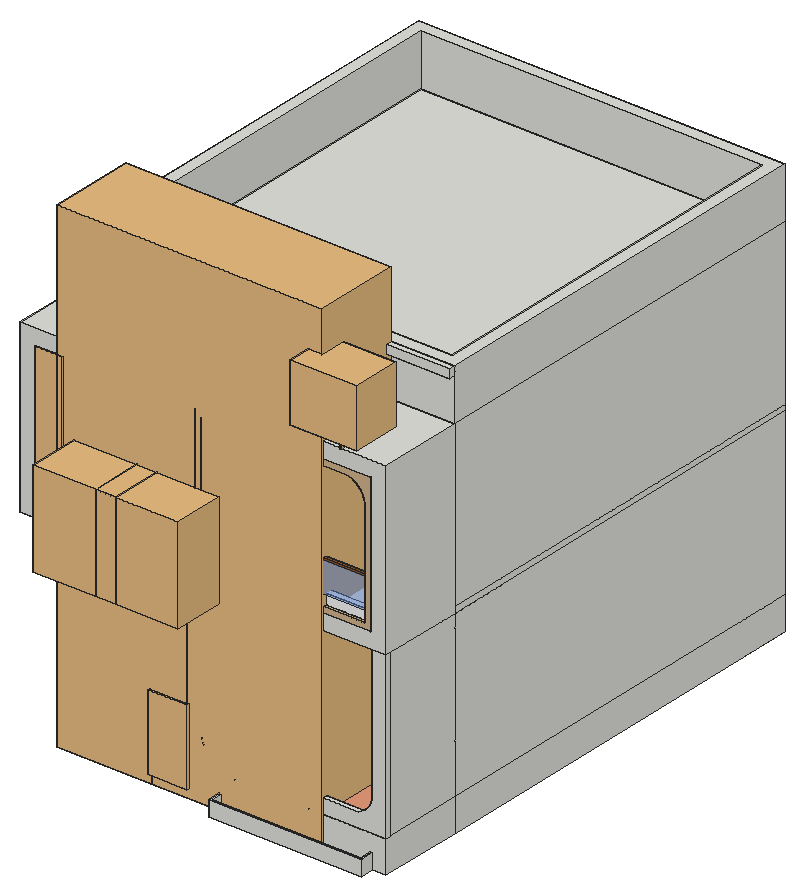
# SketchUp Ruby script. Lengths in inches.
U = 1.inch
M = Sketchup.active_model
def pt(a) = Geom::Point3d.new(a.map { |v| v * U })
def face(e, loops, mat)
  f = e.add_face(loops[0].map { |a| pt(a) })
  loops[1..].each { |l| e.add_face(l.map { |a| pt(a) }).erase! }
  f.material = f.back_material = mat if mat
  f
end
# faces: each face lists its corners as indices into pts; further lists are holes
def faces(e, pts, list, mat = nil) = list.each { |f| face(e, (f[0].is_a?(Array) ? f : [f]).map { |l| l.map { |i| pts[i] } }, mat) }
# xy, xz, yz: faces in a plane at the given z, y or x. An outline is a flat list of corners, or four numbers for a rectangle; further outlines are holes
def ring(l) = l.size == 4 ? [[l[0], l[1]], [l[2], l[1]], [l[2], l[3]], [l[0], l[3]]] : l.each_slice(2).to_a
def flat(e, list, mat, &to3) = list.each { |f| face(e, (f[0].is_a?(Array) ? f : [f]).map { |l| ring(l).map { |u, v| to3.(u, v) } }, mat) }
def xy(e, z, list, mat = nil) = flat(e, list, mat) { |x, y| [x, y, z] }
def xz(e, y, list, mat = nil) = flat(e, list, mat) { |x, z| [x, y, z] }
def yz(e, x, list, mat = nil) = flat(e, list, mat) { |y, z| [x, y, z] }
def lines(e, pts, list) = list.each { |a, b| e.add_line(pt(pts[a]), pt(pts[b])) }
# prism: a flat outline (further loops are holes) pulled along v
def prism(e, loops, v, mat = nil)
  f = face(e, loops, mat); d = Geom::Vector3d.new(v.map { |x| x * U })
  f.pushpull(f.normal.samedirection?(d) ? d.length : -d.length)
end
def box(e, o, s, mat = nil) = prism(e, [[o, [o[0] + s[0], o[1], o[2]], [o[0] + s[0], o[1] + s[1], o[2]], [o[0], o[1] + s[1], o[2]]]], [0, 0, s[2]], mat)
def at(x, y, z, deg = 0) = Geom::Transformation.translation(pt([x, y, z])) * Geom::Transformation.rotation(ORIGIN, Z_AXIS, deg.degrees)
def axes(o, x, y, z) = Geom::Transformation.new([*x, 0, *y, 0, *z, 0, *pt(o).to_a, 1])
def part(name) = M.definitions.add(name)
# library, detail: a bought-in or finely detailed component or shape, given as its bounding box
def library(name, o, s) = part(name).tap { |d| box(d.entities, o, s) }
def detail(e, o, s) = box(e.add_group.entities, o, s)
def put(e, d, t, mat = nil) = e.add_instance(d, t).tap { |i| i.material = mat if mat }
def group(e, t, mat = nil) = e.add_group.tap { |g| g.transformation = t; g.material = mat if mat }.entities
root = M.entities
M.materials.add("Heather_Skin").color = [229, 155, 121]
M.materials.add("[0035_Tan]").color = [210, 180, 140]
M.materials.add("[0128_White]").color = [255, 255, 255]
M.materials["[0128_White]"].alpha = 0.85
M.materials.add("[0129_WhiteSmoke]").color = [245, 245, 245]
M.materials.add("[Color M09]").color = [0, 0, 0]
M.materials.add("[Translucent Glass Blue]").color = [100, 149, 237]
M.materials["[Translucent Glass Blue]"].alpha = 0.5
M.materials.add("[Wood Cherry Original]").color = [152, 86, 42]
c1 = library("Rose+Jali+Design",[0,0,0],[20,1,36])
c2 = library("Hanging plant cluster",[-9.08,-12.96,-0.71],[50.92,60.22,69.94])
c3 = library("Door+01",[0,-2.84,-4],[33.31,7.1,94])
c4 = library("Window with transom",[0,0,0],[5.2,55.12,70.87])
c5 = part("Divided light sash")
xy(c5.entities,0,[[[0,-7,18,20],[1,-5,17,19]]])
xy(c5.entities,0.25,[[8.75,-5,8.75,6.75,1,6.75,1,7.25,8.75,7.25,8.75,19,9.25,19,9.25,7.25,17,7.25,17,6.75,9.25,6.75,9.25,-5]])
xy(c5.entities,0.5,[[1,-5,8.75,6.75],[9.25,-5,17,6.75],[1,7.25,8.75,19],[9.25,7.25,17,19]])
xy(c5.entities,0.75,[[8.75,-5,9.25,-5,9.25,6.75,17,6.75,17,7.25,9.25,7.25,9.25,19,8.75,19,8.75,7.25,1,7.25,1,6.75,8.75,6.75]])
xy(c5.entities,1,[[[0,-7,18,20],[1,-5,17,19]]])
xz(c5.entities,-7,[[0,0,18,1]])
xz(c5.entities,-5,[[1,0,1,0.5,8.75,0.5,8.75,0.25,9.25,0.25,9.25,0.5,17,0.5,17,0],[8.75,0.25,9.25,0.75],[1,0.5,1,1,17,1,17,0.5,9.25,0.5,9.25,0.75,8.75,0.75,8.75,0.5]])
xz(c5.entities,6.75,[[1,0.25,8.75,0.5],[9.25,0.25,17,0.5],[1,0.5,8.75,0.75],[9.25,0.5,17,0.75]])
xz(c5.entities,7.25,[[1,0.25,8.75,0.5],[9.25,0.25,17,0.5],[1,0.5,8.75,0.75],[9.25,0.5,17,0.75]])
xz(c5.entities,19,[[1,0,17,0,17,0.5,9.25,0.5,9.25,0.25,8.75,0.25,8.75,0.5,1,0.5],[8.75,0.25,9.25,0.75],[1,0.5,8.75,0.5,8.75,0.75,9.25,0.75,9.25,0.5,17,0.5,17,1,1,1]])
xz(c5.entities,20,[[0,0,18,1]])
yz(c5.entities,0,[[-7,0,20,1]])
yz(c5.entities,1,[[-5,0,19,0,19,0.5,7.25,0.5,7.25,0.25,6.75,0.25,6.75,0.5,-5,0.5],[6.75,0.25,7.25,0.75],[-5,0.5,6.75,0.5,6.75,0.75,7.25,0.75,7.25,0.5,19,0.5,19,1,-5,1]])
yz(c5.entities,8.75,[[-5,0.25,6.75,0.5],[7.25,0.25,19,0.5],[-5,0.5,6.75,0.75],[7.25,0.5,19,0.75]])
yz(c5.entities,9.25,[[-5,0.25,6.75,0.5],[7.25,0.25,19,0.5],[-5,0.5,6.75,0.75],[7.25,0.5,19,0.75]])
yz(c5.entities,17,[[-5,0,-5,0.5,6.75,0.5,6.75,0.25,7.25,0.25,7.25,0.5,19,0.5,19,0],[6.75,0.25,7.25,0.75],[-5,0.5,-5,1,19,1,19,0.5,7.25,0.5,7.25,0.75,6.75,0.75,6.75,0.5]])
yz(c5.entities,18,[[-7,0,20,1]])
c6 = part("Double-hung window 69 in. x 58 in. triple row with mullions")
xy(c6.entities,-2.625,[[[1.5,1.5,60.5,56.5],[22,2.5,40,55.5],[2.5,2.5,20.5,55.5],[41.5,2.5,59.5,55.5]]])
xy(c6.entities,0,[[[0,0,62,58],[1.5,1.5,60.5,56.5]],[1.5,1.5,60.5,2.5],[1.5,2.5,2,2.5,2,56,60,56,60,2.5,60.5,2.5,60.5,56.5,1.5,56.5],[21,2.5,21.5,56],[40.5,2.5,41,56]])
xy(c6.entities,1,[[[0,0,62,58],[1.5,2,60.5,56.5]]])
xz(c6.entities,0,[[0,0,62,1]])
xz(c6.entities,1.5,[[1.5,-2.625,60.5,0]])
xz(c6.entities,2.5,[[2.5,-2.625,2.5,-0.5,2,0,21,0,20.5,-0.5,20.5,-2.625],[22,-2.625,22,-0.5,21.5,0,40.5,0,40,-0.5,40,-2.625],[41.5,-2.625,41.5,-0.5,41,0,60,0,59.5,-0.5,59.5,-2.625]])
xz(c6.entities,55.5,[[2.5,-2.625,20.5,-0.5],[22,-2.625,40,-0.5],[41.5,-2.625,59.5,-0.5]])
xz(c6.entities,56.5,[[1.5,-2.625,60.5,0],[1.5,0,60.5,1]])
xz(c6.entities,58,[[0,0,62,1]])
yz(c6.entities,0,[[0,0,58,1]])
yz(c6.entities,1.5,[[1.5,-2.625,56.5,0],[1.5,0,2.5,0,2,1],[2.5,0,56.5,0,56.5,1,2,1]])
yz(c6.entities,2.5,[[2.5,-2.625,55.5,-0.5]])
yz(c6.entities,20.5,[[2.5,-2.625,55.5,-0.5]])
yz(c6.entities,22,[[2.5,-2.625,55.5,-0.5]])
yz(c6.entities,40,[[2.5,-2.625,55.5,-0.5]])
yz(c6.entities,41.5,[[2.5,-2.625,55.5,-0.5]])
yz(c6.entities,59.5,[[2.5,-2.625,55.5,-0.5]])
yz(c6.entities,60.5,[[1.5,-2.625,56.5,0],[1.5,0,2,1,2.5,0],[2.5,0,2,1,56.5,1,56.5,0]])
yz(c6.entities,62,[[0,0,58,1]])
p = [[2,2.5,0],[2.5,2.5,-0.5],[2.5,55.5,-0.5],[2,56,0],[21,2.5,0],[21,56,0],
  [20.5,55.5,-0.5],[20.5,2.5,-0.5],[22,2.5,-0.5],[22,55.5,-0.5],[21.5,56,0],[21.5,2.5,0],
  [40.5,2.5,0],[40.5,56,0],[40,55.5,-0.5],[40,2.5,-0.5],[41.5,2.5,-0.5],[41.5,55.5,-0.5],
  [41,56,0],[41,2.5,0],[60,56,0],[59.5,55.5,-0.5],[59.5,2.5,-0.5],[60,2.5,0],
  [60.5,1.5,0],[1.5,1.5,0],[1.5,2,1],[60.5,2,1],[60.5,2.5,0],[1.5,2.5,0]]
faces(c6.entities,p,[[0,1,2,3],[4,5,6,7],[8,9,10,11],[12,13,14,15],[16,17,18,19],[20,21,22,23],[2,6,5,3],[9,14,13,10],
  [20,18,17,21],[24,25,26,27],[27,28,23,19,12,11,4,0,29,26]])
put(c6.entities,c5,at(20.5,48.5,-1.5,180))
put(c6.entities,c5,at(2.5,9.5,-2.5))
put(c6.entities,c5,at(41.5,9.5,-2.5))
put(c6.entities,c5,at(59.5,48.5,-1.5,180))
put(c6.entities,c5,at(22,9.5,-2.5))
put(c6.entities,c5,at(40,48.5,-1.5,180))
c7 = part("Double-hung window assembly")
put(c7.entities,c6,axes([2046.74,517.98,-571.2],[-3.288,0,0],[0,0,3.072],[0,2.4,0]))
c8 = library("Entrance door",[-0.84,0,0],[9.1,39.62,78.08])
c9 = library("Group\#33",[0,0,0],[28.42,3.15,55.45])
c10 = part("Group\#40")
prism(c10.entities,[[[3.62,0.1,0],[2.875,0,0],[2.13,0.1,0],[1.4375,0.39,0],[0.84,0.84,0],[0.39,1.4375,0],[0.1,2.13,0],[0,2.875,0],[0.1,3.62,0],[0.39,4.3125,0],[0.84,4.91,0],[1.4375,5.36,0],[2.13,5.65,0],[2.875,5.75,0],[3.62,5.65,0],[4.3125,5.36,0],[4.91,4.91,0],[5.36,4.3125,0],[5.65,3.62,0],[5.75,2.875,0],[5.65,2.13,0],[5.36,1.4375,0],[4.91,0.84,0],[4.3125,0.39,0]]],[0,0,1.75])
c11 = library("Group3\#2",[-5.89,-6.37,-1],[12.43,12.74,228.94])
c12 = library("Group4\#2",[-105.05,-86.73,79.56],[214.66,175.02,286.71])
c13 = library("Group5\#2",[-160.02,-151.22,110.13],[330.59,312.52,316])
c14 = part("Group2\#2")
put(c14.entities,c11,at(0,0,0))
put(c14.entities,c12,at(0,0,0))
put(c14.entities,c13,at(0,0,0))
c15 = part("Group1\#1")
put(c15.entities,c14,at(0,0,0))
c16 = part("Difference\#2")
xy(c16.entities,0,[[0,0,0,301.25,267.375,301.25,267.375,0,179.9,0,179.9,9,258.375,9,258.375,292.25,9,292.25,9,9,133.6875,9,133.6875,0]])
xy(c16.entities,51.125,[[48.68,0,108.66,9]])
xy(c16.entities,51.44,[[195.43,0,249.56,9]])
xy(c16.entities,93.625,[[133.6875,0,179.9,9]])
xy(c16.entities,105.19,[[195.43,0,249.56,9]])
xy(c16.entities,105.5625,[[48.68,0,108.66,9]])
xy(c16.entities,120,[[[0,0,267.375,301.25],[9,9,258.375,292.25]]])
xz(c16.entities,0,[[[0,0,133.6875,0,133.6875,93.625,179.9,93.625,179.9,0,267.375,0,267.375,120,0,120],[48.68,51.125,108.66,105.5625],[195.43,51.44,249.56,105.19]]])
xz(c16.entities,9,[[[9,0,9,120,258.375,120,258.375,0,179.9,0,179.9,93.625,133.6875,93.625,133.6875,0],[48.68,51.125,108.66,105.5625],[195.43,51.44,249.56,105.19]]])
xz(c16.entities,292.25,[[9,0,258.375,120]])
xz(c16.entities,301.25,[[0,0,267.375,120]])
yz(c16.entities,0,[[0,0,301.25,120]])
yz(c16.entities,9,[[9,0,292.25,120]])
yz(c16.entities,48.68,[[0,51.125,9,105.5625]])
yz(c16.entities,108.66,[[0,51.125,9,105.5625]])
yz(c16.entities,133.6875,[[0,0,9,93.625]])
yz(c16.entities,179.9,[[0,0,9,93.625]])
yz(c16.entities,195.43,[[0,51.44,9,105.19]])
yz(c16.entities,249.56,[[0,51.44,9,105.19]])
yz(c16.entities,258.375,[[9,0,292.25,120]])
yz(c16.entities,267.375,[[0,0,301.25,120]])
c17 = part("Group19\#1")
box(c17.entities,[58.52,-33.93,153.53],[82.32,2.69,1.73])
c18 = part("Group16\#1")
box(c18.entities,[58.52,-33.73,131.31],[2.36,2.36,22.22])
c19 = part("Group20\#1")
box(c19.entities,[63.375,-33.33,131.31],[0.4,1.57,22.22])
box(c19.entities,[67.24,-33.33,131.31],[0.4,1.57,22.22])
box(c19.entities,[71.11,-33.33,131.31],[0.39,1.57,22.22])
box(c19.entities,[74.98,-33.33,131.31],[0.39,1.57,22.22])
box(c19.entities,[78.85,-33.33,131.31],[0.39,1.57,22.22])
box(c19.entities,[82.71,-33.33,131.31],[0.4,1.57,22.22])
box(c19.entities,[86.58,-33.33,131.31],[0.4,1.57,22.22])
box(c19.entities,[90.45,-33.33,131.31],[0.39,1.57,22.22])
box(c19.entities,[94.32,-33.33,131.31],[0.39,1.57,22.22])
box(c19.entities,[98.1875,-33.33,131.31],[0.39,1.57,22.22])
box(c19.entities,[102.06,-33.33,131.31],[0.39,1.57,22.22])
box(c19.entities,[105.92,-33.33,131.31],[0.4,1.57,22.22])
box(c19.entities,[109.79,-33.33,131.31],[0.4,1.57,22.22])
box(c19.entities,[113.66,-33.33,131.31],[0.39,1.57,22.22])
box(c19.entities,[117.53,-33.33,131.31],[0.39,1.57,22.22])
box(c19.entities,[121.4,-33.33,131.31],[0.39,1.57,22.22])
box(c19.entities,[125.26,-33.33,131.31],[0.4,1.57,22.22])
box(c19.entities,[129.13,-33.33,131.31],[0.4,1.57,22.22])
box(c19.entities,[144.61,-33.33,131.31],[0.39,1.57,22.22])
box(c19.entities,[133.41,-33.33,131.31],[0.39,1.57,22.22])
c20 = part("Group17\#1")
box(c20.entities,[137.39,-33.48,131.22],[2.36,2.36,22.23])
c21 = library("Group\#2",[-3.8125,-32.75,-24],[193.5625,62.5625,354.5625])
c22 = part("Group8\#1")
box(c22.entities,[63.78,28.58,255.8125],[2.36,2.37,22.23])
c23 = part("Group9\#1")
box(c23.entities,[182.12,28.58,255.8125],[2.36,2.37,22.23])
c24 = part("Group11\#1")
box(c24.entities,[63.78,28.39,278.04],[120.7,2.75,1.77])
c25 = part("Group12\#1")
box(c25.entities,[68.58,28.98,255.8125],[0.4,1.57,22.23])
box(c25.entities,[72.4,28.98,255.8125],[0.39,1.57,22.23])
box(c25.entities,[76.22,28.98,255.8125],[0.39,1.57,22.23])
box(c25.entities,[80.04,28.98,255.8125],[0.39,1.57,22.23])
box(c25.entities,[83.85,28.98,255.8125],[0.4,1.57,22.23])
box(c25.entities,[87.67,28.98,255.8125],[0.39,1.57,22.23])
box(c25.entities,[91.49,28.98,255.8125],[0.39,1.57,22.23])
box(c25.entities,[95.31,28.98,255.8125],[0.39,1.57,22.23])
box(c25.entities,[99.12,28.98,255.8125],[0.4,1.57,22.23])
box(c25.entities,[102.94,28.98,255.8125],[0.39,1.57,22.23])
box(c25.entities,[106.76,28.98,255.8125],[0.39,1.57,22.23])
box(c25.entities,[110.57,28.98,255.8125],[0.4,1.57,22.23])
box(c25.entities,[114.39,28.98,255.8125],[0.4,1.57,22.23])
box(c25.entities,[118.21,28.98,255.8125],[0.39,1.57,22.23])
box(c25.entities,[122.03,28.98,255.8125],[0.39,1.57,22.23])
box(c25.entities,[125.84,28.98,255.8125],[0.4,1.57,22.23])
box(c25.entities,[129.66,28.98,255.8125],[0.4,1.57,22.23])
box(c25.entities,[133.48,28.98,255.8125],[0.39,1.57,22.23])
box(c25.entities,[137.3,28.98,255.8125],[0.39,1.57,22.23])
box(c25.entities,[141.11,28.98,255.8125],[0.4,1.57,22.23])
box(c25.entities,[144.93,28.98,255.8125],[0.39,1.57,22.23])
box(c25.entities,[148.75,28.98,255.8125],[0.39,1.57,22.23])
box(c25.entities,[152.57,28.98,255.8125],[0.39,1.57,22.23])
box(c25.entities,[156.38,28.98,255.8125],[0.4,1.57,22.23])
box(c25.entities,[160.2,28.98,255.8125],[0.39,1.57,22.23])
box(c25.entities,[164.02,28.98,255.8125],[0.39,1.57,22.23])
box(c25.entities,[167.84,28.98,255.8125],[0.39,1.57,22.23])
box(c25.entities,[171.65,28.98,255.8125],[0.4,1.57,22.23])
box(c25.entities,[175.47,28.98,255.8125],[0.39,1.57,22.23])
box(c25.entities,[179.29,28.98,255.8125],[0.39,1.57,22.23])
c26 = part("Difference\#1")
xy(c26.entities,0,[[0,0,0,301.25,267.375,301.25,267.375,0,179.9,0,179.9,9,258.375,9,258.375,292.25,9,292.25,9,9,133.6875,9,133.6875,0]])
xy(c26.entities,35.62,[[195.43,0,245.43,9]])
xy(c26.entities,35.875,[[50.37,0,113.66,9]])
xy(c26.entities,83.125,[[50.37,0,113.66,9]])
xy(c26.entities,87.94,[[195.43,0,245.43,9]])
xy(c26.entities,93.625,[[133.6875,0,179.9,9]])
xy(c26.entities,120,[[0,0,0,301.25,267.375,301.25,267.375,0,154.54,0,154.54,9,258.375,9,258.375,292.25,9,292.25,9,9,36.2,9,36.2,0]])
xy(c26.entities,151.8125,[[154.54,-4.625,267.375,0],[0,-3.625,36.2,0]])
xy(c26.entities,157.875,[[154.54,-4.625,267.375,0],[0,-3.625,36.2,-3.625,36.2,9,9,9,9,292.25,258.375,292.25,258.375,9,154.54,9,154.54,0,267.375,0,267.375,301.25,0,301.25]])
xz(c26.entities,-4.625,[[154.54,151.8125,267.375,157.875]])
xz(c26.entities,-3.625,[[0,151.8125,36.2,157.875]])
xz(c26.entities,0,[[[0,0,133.6875,0,133.6875,93.625,179.9,93.625,179.9,0,267.375,0,267.375,120,0,120],[50.37,35.875,113.66,83.125],[195.43,35.62,245.43,87.94]],[0,120,36.2,151.8125],[154.54,120,267.375,151.8125],[154.54,151.8125,267.375,157.875]])
xz(c26.entities,9,[[[9,0,9,120,258.375,120,258.375,0,179.9,0,179.9,93.625,133.6875,93.625,133.6875,0],[50.37,35.875,113.66,83.125],[195.43,35.62,245.43,87.94]],[9,120,36.2,157.875],[154.54,120,258.375,157.875]])
xz(c26.entities,292.25,[[9,0,258.375,120],[9,120,258.375,157.875]])
xz(c26.entities,301.25,[[0,0,267.375,120],[0,120,267.375,157.875]])
yz(c26.entities,0,[[0,0,301.25,120],[0,120,0,151.8125,-3.625,151.8125,-3.625,157.875,301.25,157.875,301.25,120]])
yz(c26.entities,9,[[9,0,292.25,120],[9,120,292.25,157.875]])
yz(c26.entities,36.2,[[0,120,9,151.8125],[-3.625,151.8125,9,157.875]])
yz(c26.entities,50.37,[[0,35.875,9,83.125]])
yz(c26.entities,113.66,[[0,35.875,9,83.125]])
yz(c26.entities,133.6875,[[0,0,9,93.625]])
yz(c26.entities,154.54,[[0,120,9,151.8125],[-4.625,151.8125,0,157.875],[0,151.8125,9,157.875]])
yz(c26.entities,179.9,[[0,0,9,93.625]])
yz(c26.entities,195.43,[[0,35.62,9,87.94]])
yz(c26.entities,245.43,[[0,35.62,9,87.94]])
yz(c26.entities,258.375,[[9,0,292.25,120],[9,120,292.25,157.875]])
yz(c26.entities,267.375,[[0,0,301.25,120],[0,120,301.25,157.875],[-4.625,151.8125,0,157.875]])
g1 = group(c26.entities,at(11.31,0,7.31))
box(g1,[0,-62.3125,0],[19.64,133.625,101.39])
g2 = group(c26.entities,at(36.2,0,120))
box(g2,[0,0,0],[118.34,9,11.8125])
put(g2,c22,at(-64.96,-29.77,-244))
put(g2,c23,at(-64.96,-29.77,-244))
put(g2,c24,at(-64.96,-29.77,-244))
put(g2,c25,at(-64.96,-29.77,-244))
yz(root,0,[[9.8125,120,72.125,244]])
put(root,c1,axes([11.27,9.8125,131.31],[0.99304,0,0],[0,-0.47718,0],[0,0,2.81635]))
g3 = group(root,at(0,-10.19,-24))
xy(g3,144,[[0,20.01,267.375,82.32]])
xy(g3,155.31,[[45.125,19.76,127.625,20.01],[127.625,20.01,256.07,22.51]])
xy(g3,155.31,[[11.31,20.01,45.125,20.01,45.125,27.38,256.07,27.38,256.07,82.32,11.31,82.32]],"[0128_White]")
xy(g3,166.99,[[45.125,20.01,127.625,27.38],[127.625,22.51,256.07,27.38]],"[0128_White]")
xy(g3,190.12,[[132.18,20.01,251.53,22.51]],"[Wood Cherry Original]")
xy(g3,191.67,[[132.18,20.01,251.53,22.51]],"[Wood Cherry Original]")
xy(g3,256.69,[[11.31,20.01,256.07,82.32]])
xy(g3,268,[[0,20.01,267.375,82.32]])
xz(g3,20.01,[[[0,144,267.375,268],[11.31,155.31,256.07,256.69]]])
xz(g3,20.01,[[45.125,155.31,127.625,166.99]],"[0129_WhiteSmoke]")
xz(g3,20.01,[[132.18,167.25,251.53,190.12]],"[Translucent Glass Blue]")
xz(g3,20.01,[[132.18,190.12,251.53,191.67]],"[Wood Cherry Original]")
xz(g3,22.51,[[127.625,155.31,256.07,166.99]],"[0129_WhiteSmoke]")
xz(g3,22.51,[[132.18,190.12,251.53,191.67]],"[Wood Cherry Original]")
xz(g3,27.38,[[45.125,155.31,127.625,166.99],[127.625,155.31,256.07,166.99]])
xz(g3,82.32,[[[0,144,267.375,268],[11.31,155.31,256.07,256.69]]])
yz(g3,11.31,[[20.01,155.31,82.32,256.69]])
yz(g3,45.125,[[20.01,155.31,27.38,166.99]])
yz(g3,127.625,[[20.01,155.31,22.51,166.99]])
yz(g3,132.18,[[20.01,190.12,22.51,191.67]],"[Wood Cherry Original]")
yz(g3,251.53,[[20.01,190.12,22.51,191.67]],"[Wood Cherry Original]")
yz(g3,256.07,[[20.01,155.31,20.01,256.69,82.32,256.69,82.32,155.31,27.38,155.31,27.38,166.99,22.51,166.99,22.51,155.31]])
yz(g3,267.375,[[20.01,144,82.32,268]])
p = [[31.125,52.51,118.41],[45.125,52.51,118.41],[267.375,82.32,24],[121.58,82.32,24],[121.56,82.32,24],[116.56,82.32,24],
  [111,82.32,24],[111,82.32,13.6875],[102.94,82.32,13.6875],[102.94,82.32,6.125],[96.31,82.32,6.125],[96.31,82.32,0]]
lines(g3,p,[[0,1],[2,3],[4,5],[5,6],[6,7],[7,8],[8,9],[9,10],[10,11]])
put(g3,c2,at(52.57,24.23,135.75,-90))
put(g3,c3,axes([133.28,82.45,155.14],[1.39932,0,0],[0,1.83,0],[0,0,0.9595]))
put(g3,c2,at(98.01,24.23,135.75,-90))
put(g3,c4,axes([195.39,86.18,75.39],[0,-0.98,0],[0.98268,0,0],[0,0,0.76505]))
put(g3,c4,axes([48.88,86.18,75.125],[0,-0.98,0],[1.08457,0,0],[0,0,0.76505]))
put(g3,c7,axes([-530.14,219.34,335.35],[0.315,0,0],[0,-0.26331,0],[0,0,0.26519]))
put(g3,c8,axes([133.3,89.04,24],[0.03316,-0.99945,0],[1.16936,0.03879,0],[0,0,1.19915]))
put(g3,c4,axes([195.43,82.77,183.62],[0,-0.97258,0],[0.90707,0,0],[0,0,0.76505]))
put(g3,c9,at(94.74,18.43,6.125))
g4 = group(g3,at(64.53,42.11,346.22),"[Color M09]")
put(g4,c10,at(0,0,-1.75))
g5 = group(g4,at(73.1875,0,-1.75),"[Color M09]")
prism(g5,[[[3.62,0.1,0],[2.875,0,0],[2.13,0.1,0],[1.4375,0.39,0],[0.84,0.84,0],[0.39,1.4375,0],[0.1,2.13,0],[0,2.875,0],[0.1,3.62,0],[0.39,4.3125,0],[0.84,4.91,0],[1.4375,5.36,0],[2.13,5.65,0],[2.875,5.75,0],[3.62,5.65,0],[4.3125,5.36,0],[4.91,4.91,0],[5.36,4.3125,0],[5.65,3.62,0],[5.75,2.875,0],[5.65,2.13,0],[5.36,1.4375,0],[4.91,0.84,0],[4.3125,0.39,0]]],[0,0,1.75])
put(g4,c10,at(24.4,0,-1.75))
g6 = group(g4,at(48.79,0,-1.75))
prism(g6,[[[3.62,0.1,0],[2.875,0,0],[2.13,0.1,0],[1.4375,0.39,0],[0.84,0.84,0],[0.39,1.4375,0],[0.1,2.13,0],[0,2.875,0],[0.1,3.62,0],[0.39,4.3125,0],[0.84,4.91,0],[1.4375,5.36,0],[2.13,5.65,0],[2.875,5.75,0],[3.62,5.65,0],[4.3125,5.36,0],[4.91,4.91,0],[5.36,4.3125,0],[5.65,3.62,0],[5.75,2.875,0],[5.65,2.13,0],[5.36,1.4375,0],[4.91,0.84,0],[4.3125,0.39,0]]],[0,0,1.75])
put(g4,c10,at(73.1875,0,-1.75))
put(g3,c15,axes([234.63,20.01,268],[0.14778,0,0],[0,0.11366,0],[0,0,0.13361]))
g7 = group(g3,at(63.77,42.48,256.69))
prism(g7,[[[-0.13,4.88,-2.4375],[0,3.875,-2.4375],[-0.13,2.87,-2.4375],[-0.52,1.9375,-2.4375],[-1.13,1.13,-2.4375],[-1.9375,0.52,-2.4375],[-2.87,0.13,-2.4375],[-3.875,0,-2.4375],[-4.88,0.13,-2.4375],[-5.8125,0.52,-2.4375],[-6.62,1.13,-2.4375],[-7.23,1.9375,-2.4375],[-7.62,2.87,-2.4375],[-7.75,3.875,-2.4375],[-7.62,4.88,-2.4375],[-7.23,5.8125,-2.4375],[-6.62,6.62,-2.4375],[-5.8125,7.23,-2.4375],[-4.88,7.62,-2.4375],[-3.875,7.75,-2.4375],[-2.87,7.62,-2.4375],[-1.9375,7.23,-2.4375],[-1.13,6.62,-2.4375],[-0.52,5.8125,-2.4375]]],[0,0,2.4375],"[Color M09]")
prism(g7,[[[52.93,4.88,-2.4375],[53.0625,3.875,-2.4375],[52.93,2.87,-2.4375],[52.54,1.9375,-2.4375],[51.93,1.13,-2.4375],[51.125,0.52,-2.4375],[50.19,0.13,-2.4375],[49.1875,0,-2.4375],[48.18,0.13,-2.4375],[47.25,0.52,-2.4375],[46.45,1.13,-2.4375],[45.83,1.9375,-2.4375],[45.44,2.87,-2.4375],[45.3125,3.875,-2.4375],[45.44,4.88,-2.4375],[45.83,5.8125,-2.4375],[46.45,6.62,-2.4375],[47.25,7.23,-2.4375],[48.18,7.62,-2.4375],[49.1875,7.75,-2.4375],[50.19,7.62,-2.4375],[51.125,7.23,-2.4375],[51.93,6.62,-2.4375],[52.54,5.8125,-2.4375]]],[0,0,2.4375],"[Color M09]")
g8 = group(g3,at(0,82.32,24))
xy(g8,-24,[[96.31,-62.3125,96.31,0,0,0,0,301.25,267.375,301.25,267.375,-62.3125]])
xy(g8,-17.875,[[96.31,-62.3125,102.94,0]],"Heather_Skin")
xy(g8,-10.3125,[[102.94,-62.3125,111,0]],"Heather_Skin")
xy(g8,0,[[111,-62.3125,267.375,-62.3125,267.375,301.25,0,301.25,0,0,111,0]],"Heather_Skin")
xz(g8,-62.3125,[[96.31,-24,121.56,-24,121.56,0,111,0,111,-10.3125,102.94,-10.3125,102.94,-17.875,96.31,-17.875],[121.56,-24,267.375,0]])
xz(g8,0,[[0,-24,96.31,-24,96.31,-17.875,102.94,-17.875,102.94,-10.3125,111,-10.3125,111,0,0,0]])
xz(g8,301.25,[[0,-24,267.375,0]])
yz(g8,0,[[0,-24,301.25,0]])
yz(g8,96.31,[[-62.3125,-24,0,-17.875]],"Heather_Skin")
yz(g8,102.94,[[-62.3125,-17.875,0,-10.3125]],"Heather_Skin")
yz(g8,111,[[-62.3125,-10.3125,0,0]],"Heather_Skin")
yz(g8,267.375,[[-62.3125,-24,0,0],[0,-24,301.25,0]])
g9 = group(g3,at(0,82.32,144))
box(g9,[0,0,0],[267.375,301.25,4])
g10 = group(g3,at(145.35,10.19,0))
xy(g10,1.0625,[[1.62,1.62,110.07,9.8125]])
xy(g10,10.875,[[0,0,111.6875,0,111.6875,9.8125,110.07,9.8125,110.07,1.62,1.62,1.62,1.62,9.8125,0,9.8125]])
xz(g10,0,[[0,0,111.6875,10.875]])
xz(g10,1.62,[[1.62,1.0625,110.07,10.875]])
xz(g10,9.8125,[[0,0,1.62,10.875],[1.62,0,110.07,1.0625],[110.07,0,111.6875,10.875]])
yz(g10,0,[[0,0,9.8125,10.875]])
yz(g10,1.62,[[1.62,1.0625,9.8125,10.875]])
yz(g10,110.07,[[1.62,1.0625,9.8125,10.875]])
yz(g10,111.6875,[[0,0,9.8125,10.875]])
g11 = group(g3,at(0,82.32,268))
xy(g11,0,[[0,0,267.375,301.25]])
g12 = group(g3,at(329.92,82.32,35.02))
g13 = group(g12,at(-208.33,-62.3125,-11.02))
prism(g13,[[[126.08,3,10.78],[127.34,3,11.24],[128.54,3,11.84],[129.67,3,12.55],[130.72,3,13.38],[131.68,3,14.32],[132.53,3,15.35],[133.27,3,16.47],[133.89,3,17.66],[134.37,3,18.91],[134.72,3,20.2],[134.9375,3,21.53],[135.01,3,22.87],[135.01,3,109.22],[135.01,3,120],[145.79,3,120],[145.79,3,0],[0,3,0],[0,3,120],[10.78,3,120],[10.78,3,20.87],[10.87,3,19.55],[11.13,3,18.26],[11.55,3,17.01],[12.13,3,15.83],[12.87,3,14.73],[13.74,3,13.74],[14.73,3,12.87],[15.83,3,12.13],[17.01,3,11.55],[18.26,3,11.13],[19.55,3,10.87],[20.87,3,10.78]]],[0,-3,0])
g14 = group(g3,at(267.375,23.01,24))
box(g14,[-4,0,0],[4,59.3125,120])
g15 = group(g3,at(127.65,20.01,155.31))
g16 = group(g15,at(0,0,0),"[0035_Tan]")
prism(g16,[[[128.42,0,0],[128.42,0,101.39],[0,0,101.39],[0,0,0]],[[4.53,0,96.85],[108.3,0,96.85],[110.34,0,96.72],[112.34,0,96.32],[114.27,0,95.67],[116.09,0,94.77],[117.79,0,93.63],[119.32,0,92.29],[120.67,0,90.76],[121.8,0,89.0625],[122.7,0,87.23],[123.36,0,85.3],[123.75,0,83.3],[123.89,0,81.27],[123.89,0,4.53],[13.28,0,4.53],[12.14,0,4.61],[11.02,0,4.83],[9.93,0,5.2],[8.91,0,5.71],[7.96,0,6.34],[7.1,0,7.1],[6.34,0,7.96],[5.71,0,8.91],[5.2,0,9.93],[4.83,0,11.02],[4.61,0,12.14],[4.53,0,13.28]]],[0,2.5,0])
put(g3,c16,at(0,82.32,24))
put(g3,c17,at(-13.39,53.48,35.77))
put(g3,c18,at(-13.39,53.48,35.77))
put(g3,c19,at(-13.39,53.48,35.77))
put(g3,c20,at(-13.39,53.48,35.77))
put(g3,c21,at(31.125,52.51,24),"[0035_Tan]")
put(g3,c26,at(0,82.32,148))
